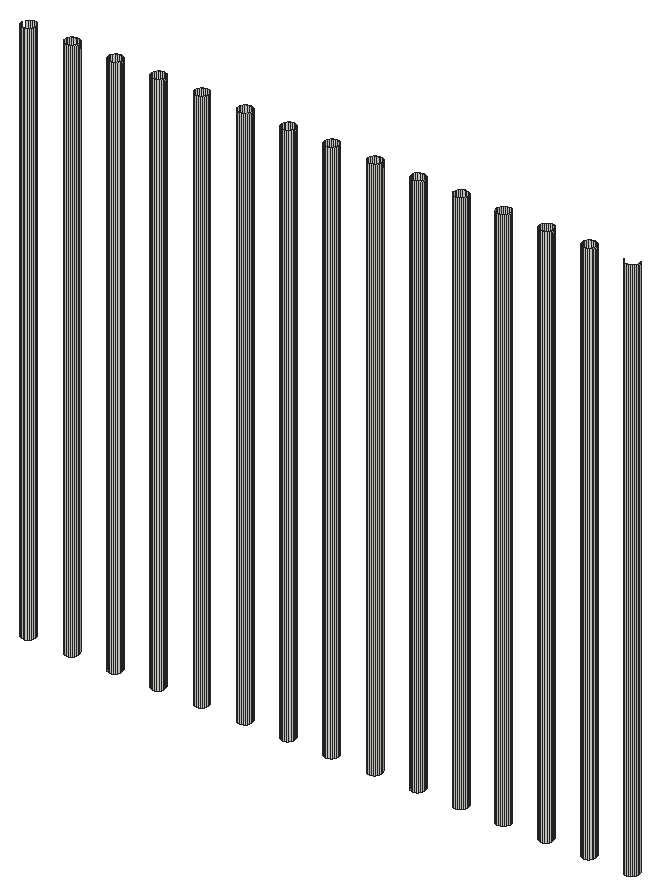
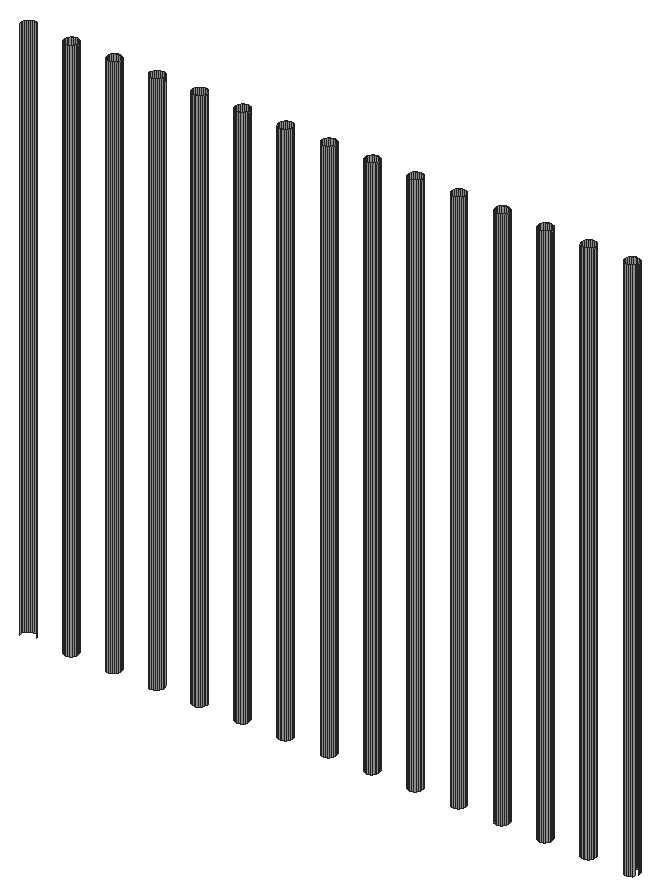
# SketchUp Ruby script. Lengths in inches.
U = 1.inch
M = Sketchup.active_model
def pt(a) = Geom::Point3d.new(a.map { |v| v * U })
def face(e, loops, mat)
  f = e.add_face(loops[0].map { |a| pt(a) })
  loops[1..].each { |l| e.add_face(l.map { |a| pt(a) }).erase! }
  f.material = f.back_material = mat if mat
  f
end
# faces: each face lists its corners as indices into pts; further lists are holes
def faces(e, pts, list, mat = nil) = list.each { |f| face(e, (f[0].is_a?(Array) ? f : [f]).map { |l| l.map { |i| pts[i] } }, mat) }
# xy, xz, yz: faces in a plane at the given z, y or x. An outline is a flat list of corners, or four numbers for a rectangle; further outlines are holes
def ring(l) = l.size == 4 ? [[l[0], l[1]], [l[2], l[1]], [l[2], l[3]], [l[0], l[3]]] : l.each_slice(2).to_a
def flat(e, list, mat, &to3) = list.each { |f| face(e, (f[0].is_a?(Array) ? f : [f]).map { |l| ring(l).map { |u, v| to3.(u, v) } }, mat) }
def xy(e, z, list, mat = nil) = flat(e, list, mat) { |x, y| [x, y, z] }
def xz(e, y, list, mat = nil) = flat(e, list, mat) { |x, z| [x, y, z] }
def yz(e, x, list, mat = nil) = flat(e, list, mat) { |y, z| [x, y, z] }
def lines(e, pts, list) = list.each { |a, b| e.add_line(pt(pts[a]), pt(pts[b])) }
# prism: a flat outline (further loops are holes) pulled along v
def prism(e, loops, v, mat = nil)
  f = face(e, loops, mat); d = Geom::Vector3d.new(v.map { |x| x * U })
  f.pushpull(f.normal.samedirection?(d) ? d.length : -d.length)
end
def box(e, o, s, mat = nil) = prism(e, [[o, [o[0] + s[0], o[1], o[2]], [o[0] + s[0], o[1] + s[1], o[2]], [o[0], o[1] + s[1], o[2]]]], [0, 0, s[2]], mat)
def at(x, y, z, deg = 0) = Geom::Transformation.translation(pt([x, y, z])) * Geom::Transformation.rotation(ORIGIN, Z_AXIS, deg.degrees)
def axes(o, x, y, z) = Geom::Transformation.new([*x, 0, *y, 0, *z, 0, *pt(o).to_a, 1])
def part(name) = M.definitions.add(name)
# library, detail: a bought-in or finely detailed component or shape, given as its bounding box
def library(name, o, s) = part(name).tap { |d| box(d.entities, o, s) }
def detail(e, o, s) = box(e.add_group.entities, o, s)
def put(e, d, t, mat = nil) = e.add_instance(d, t).tap { |i| i.material = mat if mat }
def group(e, t, mat = nil) = e.add_group.tap { |g| g.transformation = t; g.material = mat if mat }.entities
root = M.entities
p = [[409.45,133.52,409.875],[409.65,133.44,409.875],[409.65,133.44,477.08],[409.45,133.52,477.08],[409.86,133.41,409.875],[409.86,133.41,477.08],
  [410.07,133.44,409.875],[410.07,133.44,477.08],[410.26,133.52,409.875],[410.26,133.52,477.08],[414.76,133.52,409.875],[414.96,133.44,409.875],
  [414.96,133.44,477.08],[414.76,133.52,477.08],[415.17,133.41,409.875],[415.17,133.41,477.08],[415.38,133.44,409.875],[415.38,133.44,477.08],
  [415.57,133.52,409.875],[415.57,133.52,477.08],[420.07,133.52,409.875],[420.27,133.44,409.875],[420.27,133.44,477.08],[420.07,133.52,477.08],
  [420.48,133.41,409.875],[420.48,133.41,477.08],[420.69,133.44,409.875],[420.69,133.44,477.08],[420.89,133.52,409.875],[420.89,133.52,477.08],
  [425.39,133.52,409.875],[425.58,133.44,409.875],[425.58,133.44,477.08],[425.39,133.52,477.08],[425.79,133.41,409.875],[425.79,133.41,477.08],
  [426,133.44,409.875],[426,133.44,477.08],[426.2,133.52,409.875],[426.2,133.52,477.08],[430.7,133.52,409.875],[430.9,133.44,409.875],
  [430.9,133.44,477.08],[430.7,133.52,477.08],[431.11,133.41,409.875],[431.11,133.41,477.08],[431.32,133.44,409.875],[431.32,133.44,477.08],
  [431.51,133.52,409.875],[431.51,133.52,477.08],[436.01,133.52,409.875],[436.21,133.44,409.875],[436.21,133.44,477.08],[436.01,133.52,477.08],
  [436.42,133.41,409.875],[436.42,133.41,477.08],[436.63,133.44,409.875],[436.63,133.44,477.08],[436.82,133.52,409.875],[436.82,133.52,477.08],
  [441.32,133.52,409.875],[441.52,133.44,409.875],[441.52,133.44,477.08],[441.32,133.52,477.08],[441.73,133.41,409.875],[441.73,133.41,477.08],
  [441.94,133.44,409.875],[441.94,133.44,477.08],[442.14,133.52,409.875],[442.14,133.52,477.08],[446.64,133.52,409.875],[446.83,133.44,409.875],
  [446.83,133.44,477.08],[446.64,133.52,477.08],[447.04,133.41,409.875],[447.04,133.41,477.08],[447.25,133.44,409.875],[447.25,133.44,477.08],
  [447.45,133.52,409.875],[447.45,133.52,477.08],[451.95,133.52,409.875],[452.15,133.44,409.875],[452.15,133.44,477.08],[451.95,133.52,477.08],
  [452.36,133.41,409.875],[452.36,133.41,477.08],[452.57,133.44,409.875],[452.57,133.44,477.08],[452.76,133.52,409.875],[452.76,133.52,477.08],
  [457.26,133.52,409.875],[457.46,133.44,409.875],[457.46,133.44,477.08],[457.26,133.52,477.08],[457.67,133.41,409.875],[457.67,133.41,477.08],
  [457.88,133.44,409.875],[457.88,133.44,477.08],[458.07,133.52,409.875],[458.07,133.52,477.08],[462.51,133.52,409.875],[462.71,133.44,409.875],
  [462.71,133.44,477.08],[462.51,133.52,477.08],[462.92,133.41,409.875],[462.92,133.41,477.08],[463.13,133.44,409.875],[463.13,133.44,477.08],
  [463.32,133.52,409.875],[463.32,133.52,477.08],[467.76,133.52,409.875],[467.96,133.44,409.875],[467.96,133.44,477.08],[467.76,133.52,477.08],
  [468.17,133.41,409.875],[468.17,133.41,477.08],[468.38,133.44,409.875],[468.38,133.44,477.08],[468.57,133.52,409.875],[468.57,133.52,477.08],
  [473.01,133.52,409.875],[473.21,133.44,409.875],[473.21,133.44,477.08],[473.01,133.52,477.08],[473.42,133.41,409.875],[473.42,133.41,477.08],
  [473.63,133.44,409.875],[473.63,133.44,477.08],[473.82,133.52,409.875],[473.82,133.52,477.08],[478.26,133.52,409.875],[478.46,133.44,409.875],
  [478.46,133.44,477.08],[478.26,133.52,477.08],[478.67,133.41,409.875],[478.67,133.41,477.08],[478.88,133.44,409.875],[478.88,133.44,477.08],
  [479.07,133.52,409.875],[479.07,133.52,477.08],[483.51,133.52,409.875],[483.71,133.44,409.875],[483.71,133.44,477.08],[483.51,133.52,477.08],
  [483.92,133.41,409.875],[483.92,133.41,477.08],[484.13,133.44,409.875],[484.13,133.44,477.08],[484.32,133.52,409.875],[484.32,133.52,477.08],
  [409.28,133.65,409.875],[409.28,133.65,477.08],[410.43,133.65,409.875],[410.43,133.65,477.08],[414.59,133.65,409.875],[414.59,133.65,477.08],
  [415.74,133.65,409.875],[415.74,133.65,477.08],[419.91,133.65,409.875],[419.91,133.65,477.08],[421.05,133.65,409.875],[421.05,133.65,477.08],
  [425.22,133.65,409.875],[425.22,133.65,477.08],[426.37,133.65,409.875],[426.37,133.65,477.08],[430.53,133.65,409.875],[430.53,133.65,477.08],
  [431.68,133.65,409.875],[431.68,133.65,477.08],[435.84,133.65,409.875],[435.84,133.65,477.08],[436.99,133.65,409.875],[436.99,133.65,477.08],
  [441.16,133.65,409.875],[441.16,133.65,477.08],[442.3,133.65,409.875],[442.3,133.65,477.08],[446.47,133.65,409.875],[446.47,133.65,477.08],
  [447.62,133.65,409.875],[447.62,133.65,477.08],[451.78,133.65,409.875],[451.78,133.65,477.08],[452.93,133.65,409.875],[452.93,133.65,477.08],
  [457.09,133.65,409.875],[457.09,133.65,477.08],[458.24,133.65,409.875],[458.24,133.65,477.08],[462.34,133.65,409.875],[462.34,133.65,477.08],
  [463.49,133.65,409.875],[463.49,133.65,477.08],[467.59,133.65,409.875],[467.59,133.65,477.08],[468.74,133.65,409.875],[468.74,133.65,477.08],
  [472.84,133.65,409.875],[472.84,133.65,477.08],[473.99,133.65,409.875],[473.99,133.65,477.08],[478.09,133.65,409.875],[478.09,133.65,477.08],
  [479.24,133.65,409.875],[479.24,133.65,477.08],[483.34,133.65,409.875],[483.34,133.65,477.08],[484.49,133.65,409.875],[484.49,133.65,477.08],
  [409.15,133.82,409.875],[409.15,133.82,477.08],[410.56,133.82,409.875],[410.56,133.82,477.08],[414.46,133.82,409.875],[414.46,133.82,477.08],
  [415.87,133.82,409.875],[415.87,133.82,477.08],[419.78,133.82,409.875],[419.78,133.82,477.08],[421.18,133.82,409.875],[421.18,133.82,477.08],
  [425.09,133.82,409.875],[425.09,133.82,477.08],[426.5,133.82,409.875],[426.5,133.82,477.08],[430.4,133.82,409.875],[430.4,133.82,477.08],
  [431.81,133.82,409.875],[431.81,133.82,477.08],[435.71,133.82,409.875],[435.71,133.82,477.08],[437.12,133.82,409.875],[437.12,133.82,477.08],
  [441.03,133.82,409.875],[441.03,133.82,477.08],[442.43,133.82,409.875],[442.43,133.82,477.08],[446.34,133.82,409.875],[446.34,133.82,477.08],
  [447.75,133.82,409.875],[447.75,133.82,477.08],[451.65,133.82,409.875],[451.65,133.82,477.08],[453.06,133.82,409.875],[453.06,133.82,477.08],
  [456.96,133.82,409.875],[456.96,133.82,477.08],[458.37,133.82,409.875],[458.37,133.82,477.08],[462.21,133.82,409.875],[462.21,133.82,477.08],
  [463.62,133.82,409.875],[463.62,133.82,477.08],[467.46,133.82,409.875],[467.46,133.82,477.08],[468.87,133.82,409.875],[468.87,133.82,477.08],
  [472.71,133.82,409.875],[472.71,133.82,477.08],[474.12,133.82,409.875],[474.12,133.82,477.08],[477.96,133.82,409.875],[477.96,133.82,477.08],
  [479.37,133.82,409.875],[479.37,133.82,477.08],[483.21,133.82,409.875],[483.21,133.82,477.08],[484.62,133.82,409.875],[484.62,133.82,477.08],
  [409.07,134.02,409.875],[409.07,134.02,477.08],[410.64,134.02,409.875],[410.64,134.02,477.08],[414.38,134.02,409.875],[414.38,134.02,477.08],
  [415.95,134.02,409.875],[415.95,134.02,477.08],[419.7,134.02,409.875],[419.7,134.02,477.08],[421.27,134.02,409.875],[421.27,134.02,477.08],
  [425.01,134.02,409.875],[425.01,134.02,477.08],[426.58,134.02,409.875],[426.58,134.02,477.08],[430.32,134.02,409.875],[430.32,134.02,477.08],
  [431.89,134.02,409.875],[431.89,134.02,477.08],[435.63,134.02,409.875],[435.63,134.02,477.08],[437.2,134.02,409.875],[437.2,134.02,477.08],
  [440.95,134.02,409.875],[440.95,134.02,477.08],[442.52,134.02,409.875],[442.52,134.02,477.08],[446.26,134.02,409.875],[446.26,134.02,477.08],
  [447.83,134.02,409.875],[447.83,134.02,477.08],[451.57,134.02,409.875],[451.57,134.02,477.08],[453.14,134.02,409.875],[453.14,134.02,477.08],
  [456.88,134.02,409.875],[456.88,134.02,477.08],[458.45,134.02,409.875],[458.45,134.02,477.08],[462.13,134.02,409.875],[462.13,134.02,477.08],
  [463.7,134.02,409.875],[463.7,134.02,477.08],[467.38,134.02,409.875],[467.38,134.02,477.08],[468.95,134.02,409.875],[468.95,134.02,477.08],
  [472.63,134.02,409.875],[472.63,134.02,477.08],[474.2,134.02,409.875],[474.2,134.02,477.08],[477.88,134.02,409.875],[477.88,134.02,477.08],
  [479.45,134.02,409.875],[479.45,134.02,477.08],[483.13,134.02,409.875],[483.13,134.02,477.08],[484.7,134.02,409.875],[484.7,134.02,477.08],
  [409.04,134.23,409.875],[409.04,134.23,477.08],[410.67,134.23,409.875],[410.67,134.23,477.08],[414.36,134.23,409.875],[414.36,134.23,477.08],
  [415.98,134.23,409.875],[415.98,134.23,477.08],[419.67,134.23,409.875],[419.67,134.23,477.08],[421.29,134.23,409.875],[421.29,134.23,477.08],
  [424.98,134.23,409.875],[424.98,134.23,477.08],[426.61,134.23,409.875],[426.61,134.23,477.08],[430.29,134.23,409.875],[430.29,134.23,477.08],
  [431.92,134.23,409.875],[431.92,134.23,477.08],[435.61,134.23,409.875],[435.61,134.23,477.08],[437.23,134.23,409.875],[437.23,134.23,477.08],
  [440.92,134.23,409.875],[440.92,134.23,477.08],[442.54,134.23,409.875],[442.54,134.23,477.08],[446.23,134.23,409.875],[446.23,134.23,477.08],
  [447.86,134.23,409.875],[447.86,134.23,477.08],[451.54,134.23,409.875],[451.54,134.23,477.08],[453.17,134.23,409.875],[453.17,134.23,477.08],
  [456.86,134.23,409.875],[456.86,134.23,477.08],[458.48,134.23,409.875],[458.48,134.23,477.08],[462.11,134.23,409.875],[462.11,134.23,477.08],
  [463.73,134.23,409.875],[463.73,134.23,477.08],[467.36,134.23,409.875],[467.36,134.23,477.08],[468.98,134.23,409.875],[468.98,134.23,477.08],
  [472.61,134.23,409.875],[472.61,134.23,477.08],[474.23,134.23,409.875],[474.23,134.23,477.08],[477.86,134.23,409.875],[477.86,134.23,477.08],
  [479.48,134.23,409.875],[479.48,134.23,477.08],[484.73,134.23,409.875],[484.73,134.23,477.08],[410.64,134.4375,409.875],[410.64,134.4375,477.08],
  [414.38,134.4375,409.875],[414.38,134.4375,477.08],[415.95,134.4375,409.875],[415.95,134.4375,477.08],[419.7,134.4375,409.875],[419.7,134.4375,477.08],
  [421.27,134.4375,409.875],[421.27,134.4375,477.08],[425.01,134.4375,409.875],[425.01,134.4375,477.08],[426.58,134.4375,409.875],[426.58,134.4375,477.08],
  [430.32,134.4375,409.875],[430.32,134.4375,477.08],[431.89,134.4375,409.875],[431.89,134.4375,477.08],[435.63,134.4375,409.875],[435.63,134.4375,477.08],
  [437.2,134.4375,409.875],[437.2,134.4375,477.08],[440.95,134.4375,409.875],[440.95,134.4375,477.08],[442.52,134.4375,409.875],[442.52,134.4375,477.08],
  [446.26,134.4375,409.875],[446.26,134.4375,477.08],[447.83,134.4375,409.875],[447.83,134.4375,477.08],[451.57,134.4375,409.875],[451.57,134.4375,477.08],
  [453.14,134.4375,409.875],[453.14,134.4375,477.08],[456.88,134.4375,409.875],[456.88,134.4375,477.08],[458.45,134.4375,409.875],[458.45,134.4375,477.08],
  [462.13,134.4375,409.875],[462.13,134.4375,477.08],[463.7,134.4375,409.875],[463.7,134.4375,477.08],[467.38,134.4375,409.875],[467.38,134.4375,477.08],
  [468.95,134.4375,409.875],[468.95,134.4375,477.08],[472.63,134.4375,409.875],[472.63,134.4375,477.08],[474.2,134.4375,409.875],[474.2,134.4375,477.08],
  [477.88,134.4375,409.875],[477.88,134.4375,477.08],[479.45,134.4375,409.875],[479.45,134.4375,477.08],[484.7,134.4375,409.875],[484.7,134.4375,477.08],
  [410.56,134.63,409.875],[410.56,134.63,477.08],[414.46,134.63,409.875],[414.46,134.63,477.08],[415.87,134.63,409.875],[415.87,134.63,477.08],
  [419.78,134.63,409.875],[419.78,134.63,477.08],[421.18,134.63,409.875],[421.18,134.63,477.08],[425.09,134.63,409.875],[425.09,134.63,477.08],
  [426.5,134.63,409.875],[426.5,134.63,477.08],[430.4,134.63,409.875],[430.4,134.63,477.08],[431.81,134.63,409.875],[431.81,134.63,477.08],
  [435.71,134.63,409.875],[435.71,134.63,477.08],[437.12,134.63,409.875],[437.12,134.63,477.08],[441.03,134.63,409.875],[441.03,134.63,477.08],
  [442.43,134.63,409.875],[442.43,134.63,477.08],[446.34,134.63,409.875],[446.34,134.63,477.08],[447.75,134.63,409.875],[447.75,134.63,477.08],
  [451.65,134.63,409.875],[451.65,134.63,477.08],[453.06,134.63,409.875],[453.06,134.63,477.08],[456.96,134.63,409.875],[456.96,134.63,477.08],
  [458.37,134.63,409.875],[458.37,134.63,477.08],[462.21,134.63,409.875],[462.21,134.63,477.08],[463.62,134.63,409.875],[463.62,134.63,477.08],
  [467.46,134.63,409.875],[467.46,134.63,477.08],[468.87,134.63,409.875],[468.87,134.63,477.08],[472.71,134.63,409.875],[472.71,134.63,477.08],
  [474.12,134.63,409.875],[474.12,134.63,477.08],[477.96,134.63,409.875],[477.96,134.63,477.08],[479.37,134.63,409.875],[479.37,134.63,477.08],
  [484.62,134.63,409.875],[484.62,134.63,477.08],[409.28,134.8,409.875],[409.15,134.63,409.875],[409.15,134.63,477.08],[409.28,134.8,477.08],
  [410.43,134.8,409.875],[410.43,134.8,477.08],[414.59,134.8,409.875],[414.59,134.8,477.08],[415.74,134.8,409.875],[415.74,134.8,477.08],
  [419.91,134.8,409.875],[419.91,134.8,477.08],[421.05,134.8,409.875],[421.05,134.8,477.08],[425.22,134.8,409.875],[425.22,134.8,477.08],
  [426.37,134.8,409.875],[426.37,134.8,477.08],[430.53,134.8,409.875],[430.53,134.8,477.08],[431.68,134.8,409.875],[431.68,134.8,477.08],
  [435.84,134.8,409.875],[435.84,134.8,477.08],[436.99,134.8,409.875],[436.99,134.8,477.08],[441.16,134.8,409.875],[441.16,134.8,477.08],
  [442.3,134.8,409.875],[442.3,134.8,477.08],[446.47,134.8,409.875],[446.47,134.8,477.08],[447.62,134.8,409.875],[447.62,134.8,477.08],
  [451.78,134.8,409.875],[451.78,134.8,477.08],[452.93,134.8,409.875],[452.93,134.8,477.08],[457.09,134.8,409.875],[457.09,134.8,477.08],
  [458.24,134.8,409.875],[458.24,134.8,477.08],[462.34,134.8,409.875],[462.34,134.8,477.08],[463.49,134.8,409.875],[463.49,134.8,477.08],
  [467.59,134.8,409.875],[467.59,134.8,477.08],[468.74,134.8,409.875],[468.74,134.8,477.08],[472.84,134.8,409.875],[472.84,134.8,477.08],
  [473.99,134.8,409.875],[473.99,134.8,477.08],[478.09,134.8,409.875],[478.09,134.8,477.08],[479.24,134.8,409.875],[479.24,134.8,477.08],
  [409.45,134.93,409.875],[409.45,134.93,477.08],[410.26,134.93,409.875],[410.26,134.93,477.08],[414.76,134.93,409.875],[414.76,134.93,477.08],
  [415.57,134.93,409.875],[415.57,134.93,477.08],[420.07,134.93,409.875],[420.07,134.93,477.08],[420.89,134.93,409.875],[420.89,134.93,477.08],
  [425.39,134.93,409.875],[425.39,134.93,477.08],[426.2,134.93,409.875],[426.2,134.93,477.08],[430.7,134.93,409.875],[430.7,134.93,477.08],
  [431.51,134.93,409.875],[431.51,134.93,477.08],[436.01,134.93,409.875],[436.01,134.93,477.08],[436.82,134.93,409.875],[436.82,134.93,477.08],
  [441.32,134.93,409.875],[441.32,134.93,477.08],[442.14,134.93,409.875],[442.14,134.93,477.08],[446.64,134.93,409.875],[446.64,134.93,477.08],
  [447.45,134.93,409.875],[447.45,134.93,477.08],[451.95,134.93,409.875],[451.95,134.93,477.08],[452.76,134.93,409.875],[452.76,134.93,477.08],
  [457.26,134.93,409.875],[457.26,134.93,477.08],[458.07,134.93,409.875],[458.07,134.93,477.08],[462.51,134.93,409.875],[462.51,134.93,477.08],
  [463.32,134.93,409.875],[463.32,134.93,477.08],[467.76,134.93,409.875],[467.76,134.93,477.08],[468.57,134.93,409.875],[468.57,134.93,477.08],
  [473.01,134.93,409.875],[473.01,134.93,477.08],[473.82,134.93,409.875],[473.82,134.93,477.08],[478.26,134.93,409.875],[478.26,134.93,477.08],
  [479.07,134.93,409.875],[479.07,134.93,477.08],[409.65,135.01,409.875],[409.65,135.01,477.08],[410.07,135.01,409.875],[410.07,135.01,477.08],
  [414.96,135.01,409.875],[414.96,135.01,477.08],[415.38,135.01,409.875],[415.38,135.01,477.08],[420.27,135.01,409.875],[420.27,135.01,477.08],
  [420.69,135.01,409.875],[420.69,135.01,477.08],[425.58,135.01,409.875],[425.58,135.01,477.08],[426,135.01,409.875],[426,135.01,477.08],
  [430.9,135.01,409.875],[430.9,135.01,477.08],[431.32,135.01,409.875],[431.32,135.01,477.08],[436.21,135.01,409.875],[436.21,135.01,477.08],
  [436.63,135.01,409.875],[436.63,135.01,477.08],[441.52,135.01,409.875],[441.52,135.01,477.08],[441.94,135.01,409.875],[441.94,135.01,477.08],
  [446.83,135.01,409.875],[446.83,135.01,477.08],[447.25,135.01,409.875],[447.25,135.01,477.08],[452.15,135.01,409.875],[452.15,135.01,477.08],
  [452.57,135.01,409.875],[452.57,135.01,477.08],[457.46,135.01,409.875],[457.46,135.01,477.08],[457.88,135.01,409.875],[457.88,135.01,477.08],
  [462.71,135.01,409.875],[462.71,135.01,477.08],[463.13,135.01,409.875],[463.13,135.01,477.08],[467.96,135.01,409.875],[467.96,135.01,477.08],
  [468.38,135.01,409.875],[468.38,135.01,477.08],[473.21,135.01,409.875],[473.21,135.01,477.08],[473.63,135.01,409.875],[473.63,135.01,477.08],
  [478.46,135.01,409.875],[478.46,135.01,477.08],[478.88,135.01,409.875],[478.88,135.01,477.08],[409.86,135.04,409.875],[409.86,135.04,477.08],
  [415.17,135.04,409.875],[415.17,135.04,477.08],[420.48,135.04,409.875],[420.48,135.04,477.08],[425.79,135.04,409.875],[425.79,135.04,477.08],
  [431.11,135.04,409.875],[431.11,135.04,477.08],[436.42,135.04,409.875],[436.42,135.04,477.08],[441.73,135.04,409.875],[441.73,135.04,477.08],
  [447.04,135.04,409.875],[447.04,135.04,477.08],[452.36,135.04,409.875],[452.36,135.04,477.08],[457.67,135.04,409.875],[457.67,135.04,477.08],
  [462.92,135.04,409.875],[462.92,135.04,477.08],[468.17,135.04,409.875],[468.17,135.04,477.08],[473.42,135.04,409.875],[473.42,135.04,477.08],
  [478.67,135.04,409.875],[478.67,135.04,477.08]]
faces(root,p,[[0,1,2,3],[1,4,5,2],[4,6,7,5],[6,8,9,7],[10,11,12,13],[11,14,15,12],[14,16,17,15],[16,18,19,17],
  [20,21,22,23],[21,24,25,22],[24,26,27,25],[26,28,29,27],[30,31,32,33],[31,34,35,32],[34,36,37,35],[36,38,39,37],
  [40,41,42,43],[41,44,45,42],[44,46,47,45],[46,48,49,47],[50,51,52,53],[51,54,55,52],[54,56,57,55],[56,58,59,57],
  [60,61,62,63],[61,64,65,62],[64,66,67,65],[66,68,69,67],[70,71,72,73],[71,74,75,72],[74,76,77,75],[76,78,79,77],
  [80,81,82,83],[81,84,85,82],[84,86,87,85],[86,88,89,87],[90,91,92,93],[91,94,95,92],[94,96,97,95],[96,98,99,97],
  [100,101,102,103],[101,104,105,102],[104,106,107,105],[106,108,109,107],[110,111,112,113],[111,114,115,112],[114,116,117,115],[116,118,119,117],
  [120,121,122,123],[121,124,125,122],[124,126,127,125],[126,128,129,127],[130,131,132,133],[131,134,135,132],[134,136,137,135],[136,138,139,137],
  [140,141,142,143],[141,144,145,142],[144,146,147,145],[146,148,149,147],[150,0,3,151],[8,152,153,9],[154,10,13,155],[18,156,157,19],
  [158,20,23,159],[28,160,161,29],[162,30,33,163],[38,164,165,39],[166,40,43,167],[48,168,169,49],[170,50,53,171],[58,172,173,59],
  [174,60,63,175],[68,176,177,69],[178,70,73,179],[78,180,181,79],[182,80,83,183],[88,184,185,89],[186,90,93,187],[98,188,189,99],
  [190,100,103,191],[108,192,193,109],[194,110,113,195],[118,196,197,119],[198,120,123,199],[128,200,201,129],[202,130,133,203],[138,204,205,139],
  [206,140,143,207],[148,208,209,149],[210,150,151,211],[152,212,213,153],[214,154,155,215],[156,216,217,157],[218,158,159,219],[160,220,221,161],
  [222,162,163,223],[164,224,225,165],[226,166,167,227],[168,228,229,169],[230,170,171,231],[172,232,233,173],[234,174,175,235],[176,236,237,177],
  [238,178,179,239],[180,240,241,181],[242,182,183,243],[184,244,245,185],[246,186,187,247],[188,248,249,189],[250,190,191,251],[192,252,253,193],
  [254,194,195,255],[196,256,257,197],[258,198,199,259],[200,260,261,201],[262,202,203,263],[204,264,265,205],[266,206,207,267],[208,268,269,209],
  [270,210,211,271],[212,272,273,213],[274,214,215,275],[216,276,277,217],[278,218,219,279],[220,280,281,221],[282,222,223,283],[224,284,285,225],
  [286,226,227,287],[228,288,289,229],[290,230,231,291],[232,292,293,233],[294,234,235,295],[236,296,297,237],[298,238,239,299],[240,300,301,241],
  [302,242,243,303],[244,304,305,245],[306,246,247,307],[248,308,309,249],[310,250,251,311],[252,312,313,253],[314,254,255,315],[256,316,317,257],
  [318,258,259,319],[260,320,321,261],[322,262,263,323],[264,324,325,265],[326,266,267,327],[268,328,329,269],[330,270,271,331],[272,332,333,273],
  [334,274,275,335],[276,336,337,277],[338,278,279,339],[280,340,341,281],[342,282,283,343],[284,344,345,285],[346,286,287,347],[288,348,349,289],
  [350,290,291,351],[292,352,353,293],[354,294,295,355],[296,356,357,297],[358,298,299,359],[300,360,361,301],[362,302,303,363],[304,364,365,305],
  [366,306,307,367],[308,368,369,309],[370,310,311,371],[312,372,373,313],[374,314,315,375],[316,376,377,317],[378,318,319,379],[320,380,381,321],
  [382,322,323,383],[324,384,385,325],[328,386,387,329],[332,388,389,333],[390,334,335,391],[336,392,393,337],[394,338,339,395],[340,396,397,341],
  [398,342,343,399],[344,400,401,345],[402,346,347,403],[348,404,405,349],[406,350,351,407],[352,408,409,353],[410,354,355,411],[356,412,413,357],
  [414,358,359,415],[360,416,417,361],[418,362,363,419],[364,420,421,365],[422,366,367,423],[368,424,425,369],[426,370,371,427],[372,428,429,373],
  [430,374,375,431],[376,432,433,377],[434,378,379,435],[380,436,437,381],[438,382,383,439],[384,440,441,385],[386,442,443,387],[388,444,445,389],
  [446,390,391,447],[392,448,449,393],[450,394,395,451],[396,452,453,397],[454,398,399,455],[400,456,457,401],[458,402,403,459],[404,460,461,405],
  [462,406,407,463],[408,464,465,409],[466,410,411,467],[412,468,469,413],[470,414,415,471],[416,472,473,417],[474,418,419,475],[420,476,477,421],
  [478,422,423,479],[424,480,481,425],[482,426,427,483],[428,484,485,429],[486,430,431,487],[432,488,489,433],[490,434,435,491],[436,492,493,437],
  [494,438,439,495],[440,496,497,441],[442,498,499,443],[500,501,502,503],[444,504,505,445],[506,446,447,507],[448,508,509,449],[510,450,451,511],
  [452,512,513,453],[514,454,455,515],[456,516,517,457],[518,458,459,519],[460,520,521,461],[522,462,463,523],[464,524,525,465],[526,466,467,527],
  [468,528,529,469],[530,470,471,531],[472,532,533,473],[534,474,475,535],[476,536,537,477],[538,478,479,539],[480,540,541,481],[542,482,483,543],
  [484,544,545,485],[546,486,487,547],[488,548,549,489],[550,490,491,551],[492,552,553,493],[554,494,495,555],[496,556,557,497],[558,500,503,559],
  [504,560,561,505],[562,506,507,563],[508,564,565,509],[566,510,511,567],[512,568,569,513],[570,514,515,571],[516,572,573,517],[574,518,519,575],
  [520,576,577,521],[578,522,523,579],[524,580,581,525],[582,526,527,583],[528,584,585,529],[586,530,531,587],[532,588,589,533],[590,534,535,591],
  [536,592,593,537],[594,538,539,595],[540,596,597,541],[598,542,543,599],[544,600,601,545],[602,546,547,603],[548,604,605,549],[606,550,551,607],
  [552,608,609,553],[610,554,555,611],[556,612,613,557],[614,558,559,615],[560,616,617,561],[618,562,563,619],[564,620,621,565],[622,566,567,623],
  [568,624,625,569],[626,570,571,627],[572,628,629,573],[630,574,575,631],[576,632,633,577],[634,578,579,635],[580,636,637,581],[638,582,583,639],
  [584,640,641,585],[642,586,587,643],[588,644,645,589],[646,590,591,647],[592,648,649,593],[650,594,595,651],[596,652,653,597],[654,598,599,655],
  [600,656,657,601],[658,602,603,659],[604,660,661,605],[662,606,607,663],[608,664,665,609],[666,610,611,667],[612,668,669,613],[670,614,615,671],
  [616,670,671,617],[672,618,619,673],[620,672,673,621],[674,622,623,675],[624,674,675,625],[676,626,627,677],[628,676,677,629],[678,630,631,679],
  [632,678,679,633],[680,634,635,681],[636,680,681,637],[682,638,639,683],[640,682,683,641],[684,642,643,685],[644,684,685,645],[686,646,647,687],
  [648,686,687,649],[688,650,651,689],[652,688,689,653],[690,654,655,691],[656,690,691,657],[692,658,659,693],[660,692,693,661],[694,662,663,695],
  [664,694,695,665],[696,666,667,697],[668,696,697,669]])
